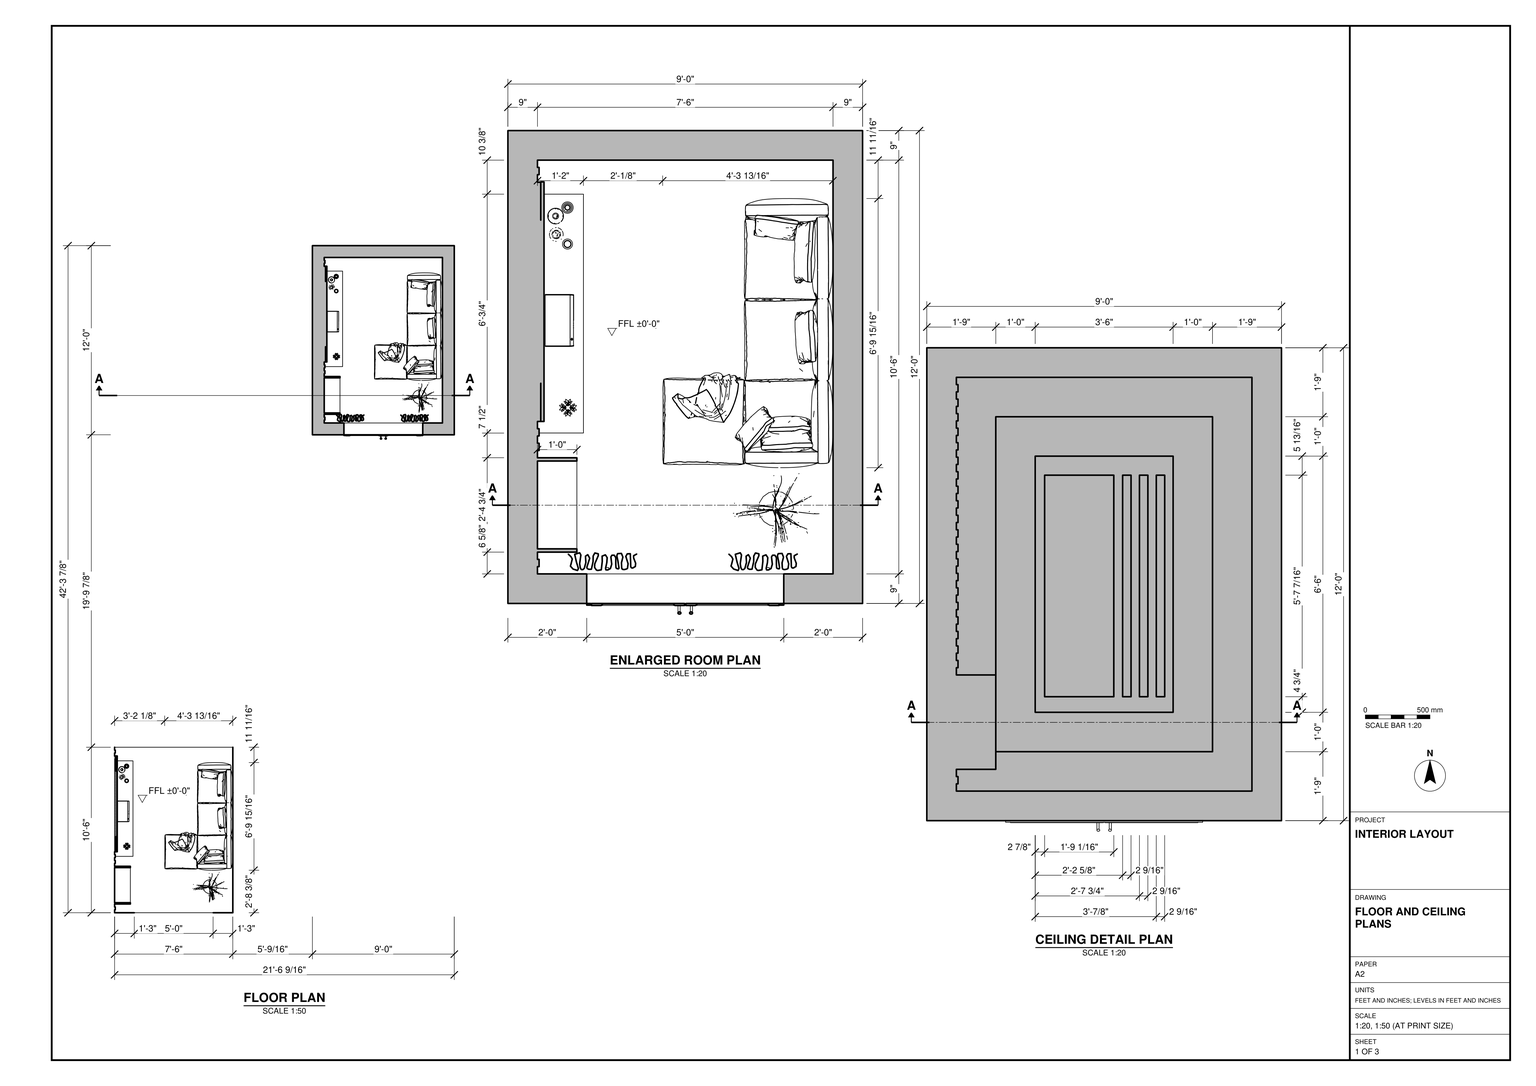
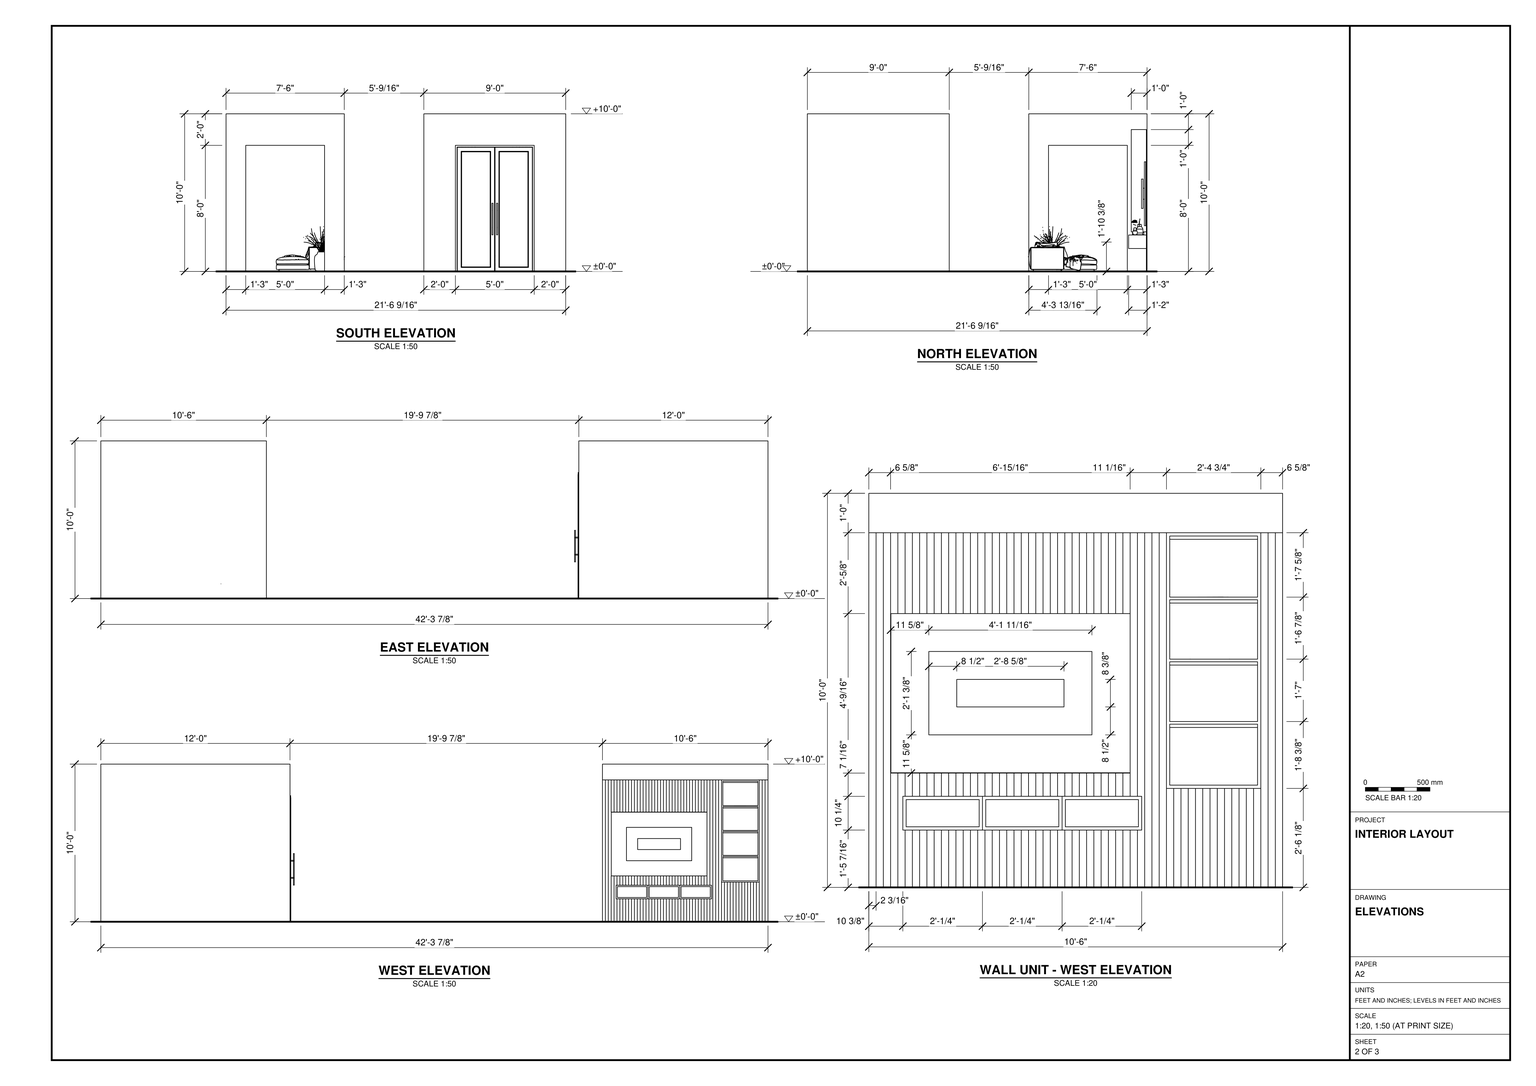
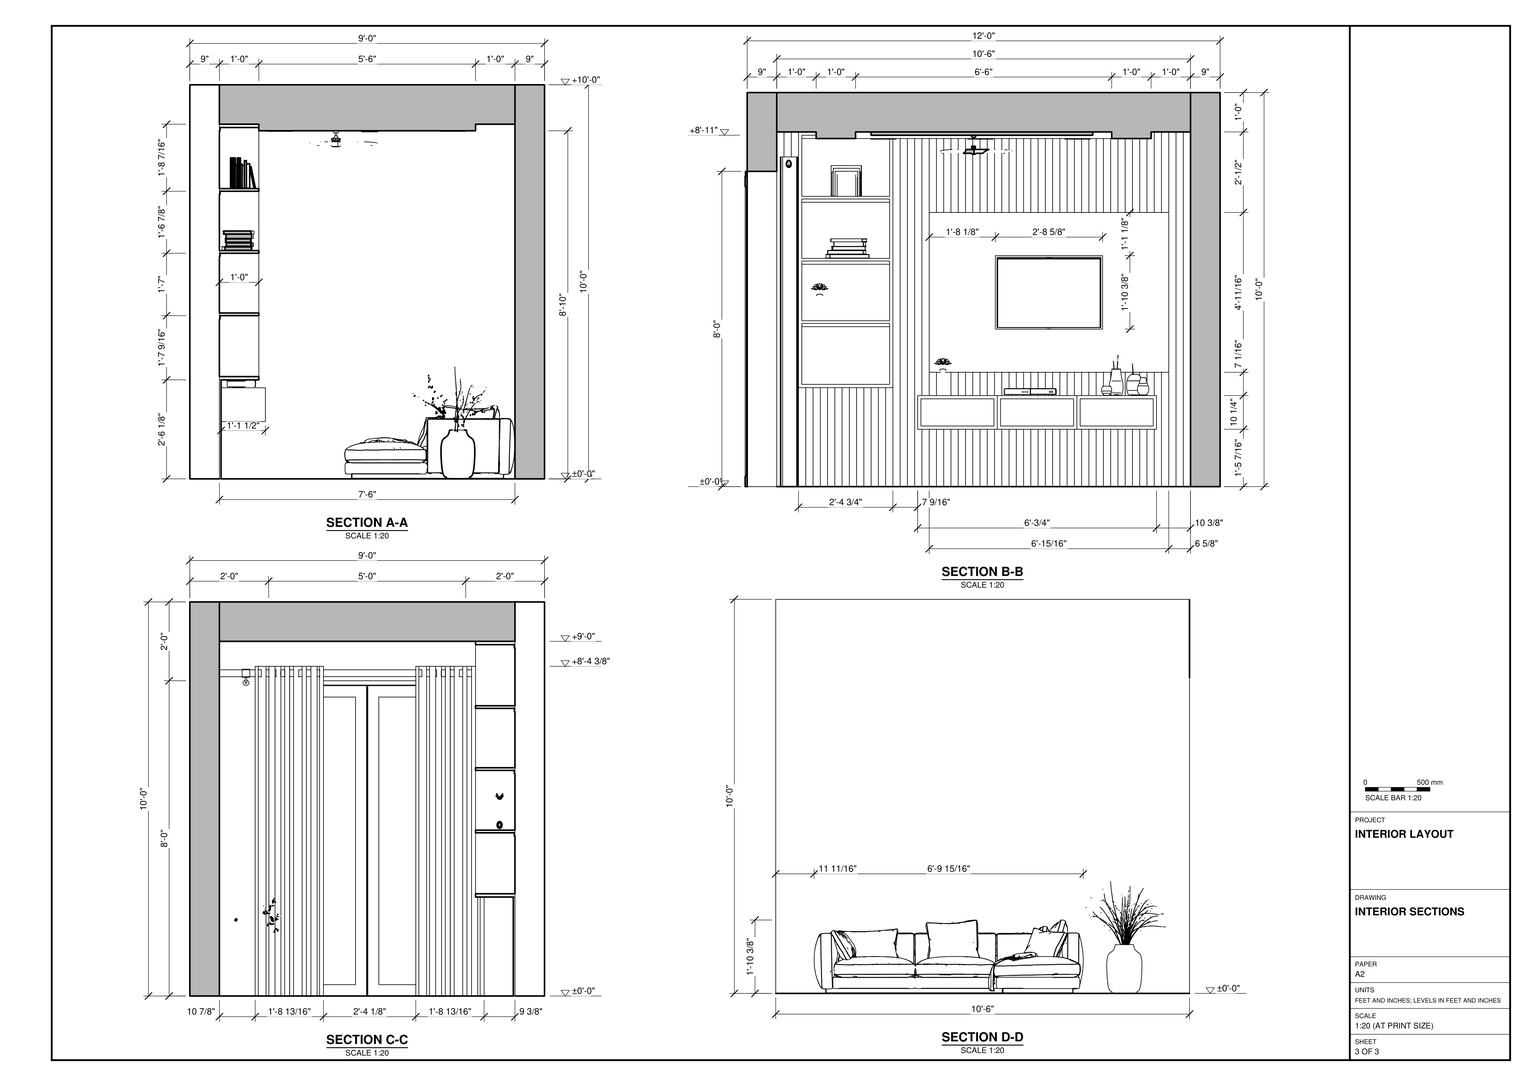
Work in feet and inches in SketchUp using task_files/diagram_01.pdf. Model both layouts shown in the floor plan: the enclosed living room to the northeast and the exposed version of its furnished interior to the southwest. Use the plan and elevations to set the gaps between them in both directions. The complete model measures 21'-6 9/16" along x, 42'-3 7/8" along y and 10'-0" along z. Set both finished floors at ±0'-0".

Build the enclosed room with a 9'-0" by 12'-0" footprint, 9" walls and a flat top. Form the stepped ceiling beneath it using the ceiling detail plan and sections. Center the paired glazed doors in the south wall and place the curtains on the room side. Fit the slatted media wall along the west side, with its screen panel, floating low cabinet and tall shelving near the doors. Place the sectional sofa opposite it with the chaise projecting toward the media wall at the south end. Include the ceiling fan, plant and shelf contents where shown. Decor and loose items may be any suitable library components.

Keep the walls, floor, roof and ceiling elements and each furniture or joinery piece in separate groups or components. Use components for repeated parts. Save one SketchUp model as output_files/furnished_living_room_and_its_exposed_interior_layout.skp.

# SketchUp Ruby script. Lengths in inches.
U = 1.inch
M = Sketchup.active_model
def pt(a) = Geom::Point3d.new(a.map { |v| v * U })
def face(e, loops, mat)
  f = e.add_face(loops[0].map { |a| pt(a) })
  loops[1..].each { |l| e.add_face(l.map { |a| pt(a) }).erase! }
  f.material = f.back_material = mat if mat
  f
end
# faces: each face lists its corners as indices into pts; further lists are holes
def faces(e, pts, list, mat = nil) = list.each { |f| face(e, (f[0].is_a?(Array) ? f : [f]).map { |l| l.map { |i| pts[i] } }, mat) }
# xy, xz, yz: faces in a plane at the given z, y or x. An outline is a flat list of corners, or four numbers for a rectangle; further outlines are holes
def ring(l) = l.size == 4 ? [[l[0], l[1]], [l[2], l[1]], [l[2], l[3]], [l[0], l[3]]] : l.each_slice(2).to_a
def flat(e, list, mat, &to3) = list.each { |f| face(e, (f[0].is_a?(Array) ? f : [f]).map { |l| ring(l).map { |u, v| to3.(u, v) } }, mat) }
def xy(e, z, list, mat = nil) = flat(e, list, mat) { |x, y| [x, y, z] }
def xz(e, y, list, mat = nil) = flat(e, list, mat) { |x, z| [x, y, z] }
def yz(e, x, list, mat = nil) = flat(e, list, mat) { |y, z| [x, y, z] }
def lines(e, pts, list) = list.each { |a, b| e.add_line(pt(pts[a]), pt(pts[b])) }
# prism: a flat outline (further loops are holes) pulled along v
def prism(e, loops, v, mat = nil)
  f = face(e, loops, mat); d = Geom::Vector3d.new(v.map { |x| x * U })
  f.pushpull(f.normal.samedirection?(d) ? d.length : -d.length)
end
def box(e, o, s, mat = nil) = prism(e, [[o, [o[0] + s[0], o[1], o[2]], [o[0] + s[0], o[1] + s[1], o[2]], [o[0], o[1] + s[1], o[2]]]], [0, 0, s[2]], mat)
def at(x, y, z, deg = 0) = Geom::Transformation.translation(pt([x, y, z])) * Geom::Transformation.rotation(ORIGIN, Z_AXIS, deg.degrees)
def axes(o, x, y, z) = Geom::Transformation.new([*x, 0, *y, 0, *z, 0, *pt(o).to_a, 1])
def part(name) = M.definitions.add(name)
# library, detail: a bought-in or finely detailed component or shape, given as its bounding box
def library(name, o, s) = part(name).tap { |d| box(d.entities, o, s) }
def detail(e, o, s) = box(e.add_group.entities, o, s)
def put(e, d, t, mat = nil) = e.add_instance(d, t).tap { |i| i.material = mat if mat }
def group(e, t, mat = nil) = e.add_group.tap { |g| g.transformation = t; g.material = mat if mat }.entities
root = M.entities
M.materials.add("Iron_Blurry_5cm\#1").color = [36, 36, 36]
M.materials.add("Teddy_Shoes").color = [254, 255, 169]
M.materials.add("[Wood Veneer 01]").color = [120, 70, 37]
c1 = library("RIDEAUX \#16",[0,0,0],[103.86,7.74,93.57])
c2 = library("Furnished living room",[0,-0.13,0],[93.45,126.13,120])
c3 = library("Door panel",[0.25,-5.22,0],[34,5.22,109.34])
c4 = library("Avation+Styled+Ceiling+Fan_JSB",[-19.77,-29.63,-13.8125],[51.59,58.16,13.8125])
c5 = library("Group\#3",[-53.48,-11.77,-2],[60.44,109.85,2.2])
xy(root,0,[[0,0.5,0,144.5,108,144.5,108,0.5,84,0.5,84,9.5,99,9.5,99,135.5,9,135.5,9,9.5,24,9.5,24,0.5]])
xy(root,96,[[24,0.5,84,9.5]])
xy(root,120,[[[0,0.5,108,144.5],[9,9.5,99,135.5]]])
xz(root,0.5,[[0,0,24,0,24,96,84,96,84,0,108,0,108,120,0,120]])
xz(root,135.5,[[9,0,99,120]])
xz(root,144.5,[[0,0,108,120]])
yz(root,0,[[0.5,0,144.5,120]])
yz(root,24,[[0.5,0,9.5,96]])
yz(root,84,[[0.5,0,9.5,96]])
yz(root,108,[[0.5,0,144.5,120]])
put(root,c1,axes([9,10.54,0],[0.86658,0,0],[0,0.69748,0],[0,0,1.07294]))
put(root,c2,at(9,9.5,0))
put(root,c2,at(-150.58,-363.34,0))
g1 = group(root,at(24,0.5,0))
prism(g1,[[[1.25,0,0],[0,0,0],[0,0,96],[60,0,96],[60,0,0],[58.75,0,0],[58.75,0,94.7],[30,0,94.7],[1.25,0,94.7]]],[0,-0.5,0],"Iron_Blurry_5cm\#1")
p = [[30,0,0],[1.25,0,0],[30,0,94.7]]
lines(g1,p,[[0,1],[2,0]])
put(g1,c3,axes([30,0,0],[0.83333,0,0],[0,0.62,0],[0,0,0.86413]),"Iron_Blurry_5cm\#1")
put(g1,c3,axes([30,0,0],[-0.83333,0,0],[0,0.62,0],[0,0,0.86413]),"Iron_Blurry_5cm\#1")
g2 = group(root,at(9,9.5,120))
xy(g2,-14,[[[12,12,78,114],[24,24,66,102]]])
xy(g2,-13,[[26.875,28.74,47.9375,96.21],[50.625,28.74,53.1875,96.21],[55.75,28.74,58.3125,96.21],[60.875,28.74,63.4375,96.21]],"[Wood Veneer 01]")
xy(g2,-12,[[[0,0,90,126],[12,12,78,114]],[[24,24,66,102],[26.875,28.74,47.9375,96.21],[60.875,28.74,63.4375,96.21],[55.75,28.74,58.3125,96.21],[50.625,28.74,53.1875,96.21]],[26.875,28.74,47.9375,96.21]])
xy(g2,-11.3125,[[60.875,24,63.4375,102]])
xy(g2,-9.3125,[[60.875,24,63.4375,102]])
xy(g2,0,[[0,0,90,126]])
xz(g2,0,[[0,-12,90,0]])
xz(g2,12,[[12,-14,78,-12]])
xz(g2,24,[[24,-14,66,-12],[60.875,-12,63.4375,-11.3125],[60.875,-11.3125,63.4375,-9.3125]])
xz(g2,28.74,[[26.875,-13,47.9375,-12],[50.625,-13,53.1875,-12],[55.75,-13,58.3125,-12],[60.875,-13,63.4375,-12]],"Teddy_Shoes")
xz(g2,96.21,[[26.875,-13,47.9375,-12],[50.625,-13,53.1875,-12],[55.75,-13,58.3125,-12],[60.875,-13,63.4375,-12]],"Teddy_Shoes")
xz(g2,102,[[24,-14,66,-12],[60.875,-12,63.4375,-11.3125],[60.875,-11.3125,63.4375,-9.3125]])
xz(g2,114,[[12,-14,78,-12]])
xz(g2,126,[[0,-12,90,0]])
yz(g2,0,[[0,-12,126,0]])
yz(g2,12,[[12,-14,114,-12]])
yz(g2,24,[[24,-14,102,-12]])
yz(g2,26.875,[[28.74,-13,96.21,-12]],"Teddy_Shoes")
yz(g2,47.9375,[[28.74,-13,96.21,-12]],"Teddy_Shoes")
yz(g2,50.625,[[28.74,-13,96.21,-12.5],[28.74,-12.5,96.21,-12]])
yz(g2,53.1875,[[28.74,-13,96.21,-12]],"Teddy_Shoes")
yz(g2,55.75,[[28.74,-13,96.21,-12]],"Teddy_Shoes")
yz(g2,58.3125,[[28.74,-13,96.21,-12]],"Teddy_Shoes")
yz(g2,60.875,[[24,-11.3125,102,-9.3125]])
yz(g2,60.875,[[28.74,-13,96.21,-12]],"Teddy_Shoes")
yz(g2,63.4375,[[24,-11.3125,102,-9.3125]])
yz(g2,63.4375,[[28.74,-13,96.21,-12]],"Teddy_Shoes")
yz(g2,66,[[24,-14,102,-12]])
yz(g2,78,[[12,-14,114,-12]])
yz(g2,90,[[0,-12,126,0]])
p = [[47.9375,28.84,-12.5],[47.9375,28.74,-12.5]]
lines(g2,p,[[0,1]])
put(g2,c4,axes([35.48,59.95,-13],[0.43,0,0],[0,0.43,0],[0,0,0.43]))
put(g2,c5,axes([67.95,25.84,-14],[1,0,0],[0,1,0],[0,0,-1]),"Teddy_Shoes")
